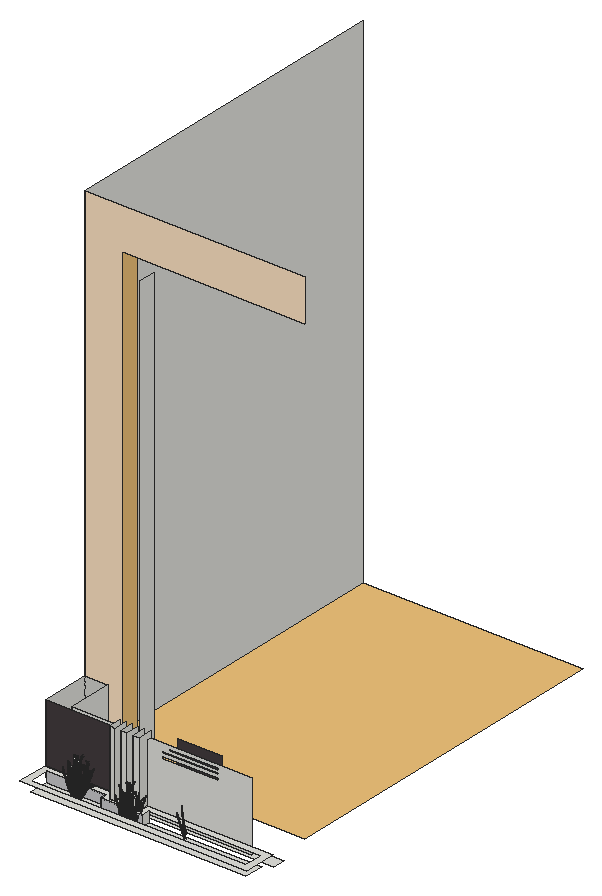
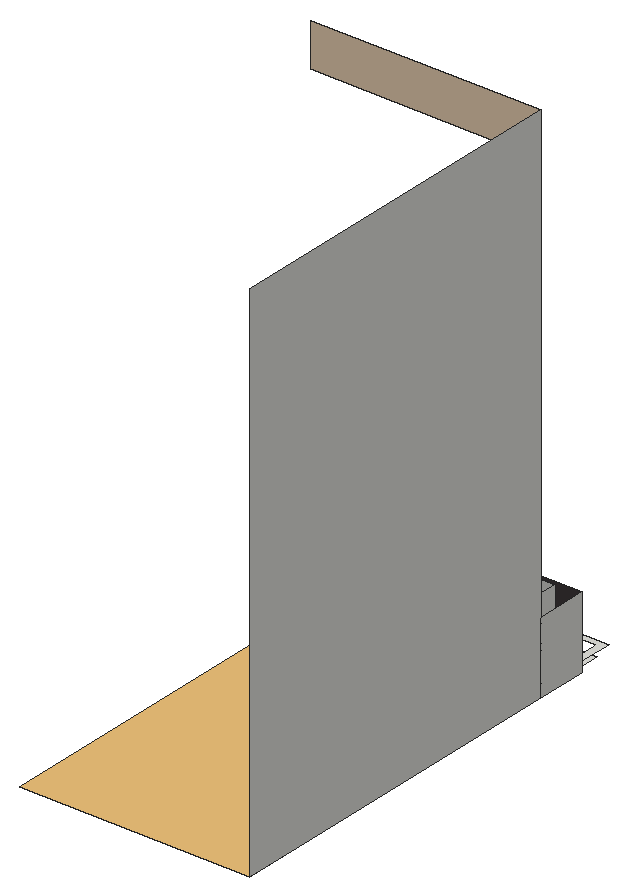
# SketchUp Ruby script. Lengths in inches.
U = 1.inch
M = Sketchup.active_model
def pt(a) = Geom::Point3d.new(a.map { |v| v * U })
def face(e, loops, mat)
  f = e.add_face(loops[0].map { |a| pt(a) })
  loops[1..].each { |l| e.add_face(l.map { |a| pt(a) }).erase! }
  f.material = f.back_material = mat if mat
  f
end
# faces: each face lists its corners as indices into pts; further lists are holes
def faces(e, pts, list, mat = nil) = list.each { |f| face(e, (f[0].is_a?(Array) ? f : [f]).map { |l| l.map { |i| pts[i] } }, mat) }
# xy, xz, yz: faces in a plane at the given z, y or x. An outline is a flat list of corners, or four numbers for a rectangle; further outlines are holes
def ring(l) = l.size == 4 ? [[l[0], l[1]], [l[2], l[1]], [l[2], l[3]], [l[0], l[3]]] : l.each_slice(2).to_a
def flat(e, list, mat, &to3) = list.each { |f| face(e, (f[0].is_a?(Array) ? f : [f]).map { |l| ring(l).map { |u, v| to3.(u, v) } }, mat) }
def xy(e, z, list, mat = nil) = flat(e, list, mat) { |x, y| [x, y, z] }
def xz(e, y, list, mat = nil) = flat(e, list, mat) { |x, z| [x, y, z] }
def yz(e, x, list, mat = nil) = flat(e, list, mat) { |y, z| [x, y, z] }
def lines(e, pts, list) = list.each { |a, b| e.add_line(pt(pts[a]), pt(pts[b])) }
# prism: a flat outline (further loops are holes) pulled along v
def prism(e, loops, v, mat = nil)
  f = face(e, loops, mat); d = Geom::Vector3d.new(v.map { |x| x * U })
  f.pushpull(f.normal.samedirection?(d) ? d.length : -d.length)
end
def box(e, o, s, mat = nil) = prism(e, [[o, [o[0] + s[0], o[1], o[2]], [o[0] + s[0], o[1] + s[1], o[2]], [o[0], o[1] + s[1], o[2]]]], [0, 0, s[2]], mat)
def at(x, y, z, deg = 0) = Geom::Transformation.translation(pt([x, y, z])) * Geom::Transformation.rotation(ORIGIN, Z_AXIS, deg.degrees)
def axes(o, x, y, z) = Geom::Transformation.new([*x, 0, *y, 0, *z, 0, *pt(o).to_a, 1])
def part(name) = M.definitions.add(name)
# library, detail: a bought-in or finely detailed component or shape, given as its bounding box
def library(name, o, s) = part(name).tap { |d| box(d.entities, o, s) }
def detail(e, o, s) = box(e.add_group.entities, o, s)
def put(e, d, t, mat = nil) = e.add_instance(d, t).tap { |i| i.material = mat if mat }
def group(e, t, mat = nil) = e.add_group.tap { |g| g.transformation = t; g.material = mat if mat }.entities
root = M.entities
M.materials.add("[0012_Bisque]").color = [255, 228, 196]
M.materials.add("[Asphalt New]").color = [67, 60, 62]
M.materials.add("[Polished Concrete New]").color = [200, 200, 203]
M.materials.add("[Wood OSB]").color = [240, 195, 122]
c1 = part("fur_instance\#8")
p = [[-0.25,1.49,0.03],[0.25,-1.49,-0.03],[0.44,-1.47,1.51],[-0.05,1.47,1.57],[0.65,-1.44,3.05],[0.16,1.45,3.11],
  [0.86,-1.42,4.59],[0.38,1.44,4.65],[1.1,-1.39,6.13],[0.62,1.43,6.18],[1.34,-1.35,7.66],[0.875,1.42,7.72],
  [1.6,-1.32,9.19],[1.14,1.41,9.25],[1.88,-1.28,10.72],[1.43,1.41,10.78],[2.18,-1.24,12.25],[1.73,1.41,12.3],
  [2.49,-1.19,13.77],[2.05,1.41,13.82],[2.83,-1.15,15.29],[2.4,1.41,15.34],[3.18,-1.09,16.8],[2.76,1.42,16.85],
  [3.56,-1.03,18.31],[3.14,1.43,18.35],[3.96,-0.97,19.81],[3.55,1.44,19.85],[4.38,-0.91,21.3],[3.99,1.46,21.35],
  [4.84,-0.83,22.78],[4.45,1.48,22.83],[5.32,-0.76,24.26],[4.93,1.51,24.31],[5.82,-0.67,25.73],[5.45,1.54,25.77],
  [6.36,-0.59,27.18],[6,1.57,27.23],[6.93,-0.49,28.625],[6.58,1.61,28.67],[7.54,-0.39,30.05],[7.19,1.66,30.1],
  [8.18,-0.28,31.47],[7.84,1.71,31.51],[8.85,-0.16,32.86],[8.53,1.77,32.9],[9.57,-0.04,34.24],[9.25,1.83,34.27],
  [10.32,0.09,35.59],[10.02,1.9,35.625],[11.12,0.23,36.92],[10.82,1.97,36.95],[11.95,0.38,38.22],[11.67,2.06,38.25],
  [12.84,0.54,39.49],[12.57,2.14,39.52],[13.76,0.71,40.73],[13.51,2.24,40.76],[14.73,0.89,41.93],[14.49,2.34,41.95],
  [15.75,1.08,43.09],[15.52,2.45,43.11],[16.82,1.28,44.2],[16.6,2.5625,44.23],[17.93,1.5,45.27],[17.73,2.68,45.29],
  [19.08,1.73,46.28],[18.9,2.81,46.3],[20.29,1.97,47.24],[20.125,2.93,47.26],[21.53,2.22,48.13],[21.39,3.0625,48.15],
  [22.82,2.5,48.96],[22.7,3.1875,48.98],[24.14,2.8125,49.72],[24.06,3.3,49.73],[25.48,3.27,50.41]]
faces(c1.entities,p,[[0,1,2,3],[3,2,4,5],[5,4,6,7],[7,6,8,9],[9,8,10,11],[11,10,12,13],[13,12,14,15],[15,14,16,17],
  [17,16,18,19],[19,18,20,21],[21,20,22,23],[23,22,24,25],[25,24,26,27],[27,26,28,29],[29,28,30,31],[31,30,32,33],
  [33,32,34,35],[35,34,36,37],[37,36,38,39],[39,38,40,41],[41,40,42,43],[43,42,44,45],[45,44,46,47],[47,46,48,49],
  [49,48,50,51],[51,50,52,53],[53,52,54,55],[55,54,56,57],[57,56,58,59],[59,58,60,61],[61,60,62,63],[63,62,64,65],
  [65,64,66,67],[67,66,68,69],[69,68,70,71],[71,70,72,73],[73,72,74,75],[75,74,76]])
xy(root,0,[[11.52,60.29,230.42,60.29,230.42,79.88,115.35,79.88,115.35,73.19,72.16,73.19,72.16,79.88,11.52,79.88],[78.43,76.52,84.2,86.15],[89.84,76.52,96.33,86.15],[102.45,76.52,109.08,86.15],[5.25,86.15,238.24,86.15,238.24,98.26,211.95,98.26,211.95,90.32,28.64,90.32,28.64,136.77,5.25,136.77],
  [43.27,136.77,60.84,154.83]])
xy(root,0,[[5.25,136.77,43.27,136.77,43.27,154.83,60.84,154.83,60.84,136.77,228.75,136.77,228.75,490.875,5.25,490.875]],"[Wood OSB]")
xy(root,10.375,[[[5.25,54.02,236.6875,54.02,236.6875,86.15,109.08,86.15,109.08,76.52,102.45,76.52,102.45,86.15,96.33,86.15,96.33,76.52,89.84,76.52,89.84,86.15,84.2,86.15,84.2,76.52,78.43,76.52,78.43,86.15,5.25,86.15],[11.52,60.29,11.52,79.88,72.16,79.88,72.16,73.19,115.35,73.19,115.35,79.88,230.42,79.88,230.42,60.29]]])
xz(root,73.19,[[72.16,0,90.47,10.375],[90.47,0,102.6,10.375],[102.6,0,115.35,10.375]],"[Polished Concrete New]")
xz(root,76.52,[[78.43,0,84.2,10.375],[89.84,0,96.33,10.375],[102.45,0,109.08,10.375],[78.43,10.375,84.2,76.5625],[89.84,10.375,96.33,76.5625],
  [102.45,10.375,109.08,76.5625]])
xz(root,79.88,[[11.52,0,72.16,10.375]],"[Polished Concrete New]")
xz(root,86.15,[[5.25,0,78.43,10.375],[84.2,0,89.84,10.375],[96.33,0,102.45,10.375]])
xz(root,86.15,[[5.25,10.375,78.43,70.5625],[84.2,10.375,89.84,70.5625],[96.33,10.375,102.45,70.5625]],"[Asphalt New]")
xz(root,90.32,[[[28.64,0,211.95,70.5625],[120.75,55.78,178.5,58.72],[120.5,60.82,178.5,63.13],[127.31,64.89,178.5,67.33]]])
xz(root,136.77,[[28.64,0,43.27,0,43.27,470.41,228.75,470.41,228.75,513.13,5.25,513.13,5.25,70.5625,28.64,70.5625]],"[0012_Bisque]")
xz(root,136.77,[[99.93,0,144.79,46.08]],"[Asphalt New]")
yz(root,5.25,[[86.15,0,136.77,70.5625],[136.77,0,490.875,513.13]])
yz(root,28.64,[[90.32,0,136.77,70.5625]])
yz(root,43.27,[[136.77,0,154.83,470.41]],"[Wood OSB]")
yz(root,60.84,[[136.77,0,154.83,450.1]])
yz(root,72.16,[[73.19,0,79.88,10.375]])
yz(root,78.43,[[76.52,0,86.15,10.375],[76.52,10.375,76.52,76.5625,90.09,76.5625,90.09,70.5625,86.15,70.5625,86.15,10.375]])
yz(root,84.2,[[76.52,0,86.15,10.375],[76.52,10.375,86.15,10.375,86.15,70.5625,90.09,70.5625,90.09,76.5625,76.52,76.5625]])
yz(root,89.84,[[76.52,0,86.15,10.375],[76.52,10.375,76.52,76.5625,90.32,76.5625,90.32,70.5625,86.15,70.5625,86.15,10.375]])
yz(root,96.33,[[76.52,0,86.15,10.375],[76.52,10.375,86.15,10.375,86.15,70.5625,90.32,70.5625,90.32,76.5625,76.52,76.5625]])
yz(root,102.45,[[76.52,0,86.15,10.375],[76.52,10.375,76.52,76.5625,90.32,76.5625,90.32,70.5625,86.15,70.5625,86.15,10.375]])
yz(root,109.08,[[76.52,0,86.15,10.375],[76.52,10.375,86.15,10.375,86.15,70.5625,90.32,70.5625,90.32,76.5625,76.52,76.5625]])
yz(root,115.35,[[73.19,0,79.88,10.375]])
put(root,c1,axes([98.37,74.84,2.3],[-0.12046,-0.19753,0.07695],[0.20061,-0.12871,0.24478],[-0.08711,0.03599,0.49657]))
put(root,c1,axes([44.62,71.44,4.95],[0.17949,0.03208,0.20009],[-0.02216,0.19765,-0.22548],[-0.11594,0.04484,0.37468]))
put(root,c1,axes([97.88,71.44,-0.97],[0.17949,0.03208,0.20009],[-0.02216,0.19765,-0.22548],[-0.11594,0.04484,0.37468]))
put(root,c1,axes([48.35,71.48,11.67],[-0.12955,0.21354,-0.0433],[-0.21401,-0.10243,0.0018],[-0.01549,-0.03509,0.55942]))
put(root,c1,axes([101.61,71.48,5.75],[-0.12955,0.21354,-0.0433],[-0.21401,-0.10243,0.0018],[-0.01549,-0.03509,0.55942]))
put(root,c1,axes([46.31,70.35,7.49],[0.00664,0.20286,-0.1262],[-0.19518,0.01818,-0.18229],[-0.08769,0.01816,0.42485]))
put(root,c1,axes([99.5625,70.35,1.57],[0.00664,0.20286,-0.1262],[-0.19518,0.01818,-0.18229],[-0.08769,0.01816,0.42485]))
put(root,c1,axes([48.88,72.47,3.5],[0.03807,-0.14827,0.33406],[0.19165,0.02974,-0.03379],[-0.02912,0.11286,0.28781]))
put(root,c1,axes([102.14,72.47,-2.42],[0.03807,-0.14827,0.33406],[0.19165,0.02974,-0.03379],[-0.02912,0.11286,0.28781]))
put(root,c1,axes([47.29,69.77,2.75],[0.10395,0.11836,-0.12851],[-0.11439,0.07411,-0.26217],[-0.07351,0.08501,0.2481]))
put(root,c1,axes([100.55,69.77,-3.17],[0.10395,0.11836,-0.12851],[-0.11439,0.07411,-0.26217],[-0.07351,0.08501,0.2481]))
put(root,c1,axes([41.98,71.41,6.21],[-0.08139,0.23064,-0.15312],[-0.1699,-0.05496,-0.32193],[-0.16391,-0.02606,0.43057]))
put(root,c1,axes([95.24,71.41,0.29],[-0.08139,0.23064,-0.15312],[-0.1699,-0.05496,-0.32193],[-0.16391,-0.02606,0.43057]))
put(root,c1,axes([158.29,71.41,5.67],[-0.08139,0.23064,-0.15312],[-0.1699,-0.05496,-0.32193],[-0.16391,-0.02606,0.43057]))
put(root,c1,axes([46.52,72.15,2.91],[0.12897,-0.08882,0.30598],[0.12311,0.13439,-0.14076],[-0.0848,0.09806,0.28618]))
put(root,c1,axes([99.78,72.15,-3.01],[0.12897,-0.08882,0.30598],[0.12311,0.13439,-0.14076],[-0.0848,0.09806,0.28618]))
put(root,c1,axes([52.9,72.82,3.01],[-0.12598,-0.09298,0.35138],[0.14548,-0.16001,0.09177],[0.09178,0.08501,0.30971]))
put(root,c1,axes([106.16,72.82,-2.91],[-0.12598,-0.09298,0.35138],[0.14548,-0.16001,0.09177],[0.09178,0.08501,0.30971]))
put(root,c1,axes([52.3,74.05,6],[0.17475,-0.1628,0.03799],[0.13362,0.1403,-0.32315],[0.08136,0.06328,0.41208]))
put(root,c1,axes([105.55,74.05,0.08],[0.17475,-0.1628,0.03799],[0.13362,0.1403,-0.32315],[0.08136,0.06328,0.41208]))
put(root,c1,axes([51.24,73.21,2.9],[-0.04728,-0.14736,0.35137],[0.1919,-0.08682,-0.02284],[0.06183,0.09936,0.30152]))
put(root,c1,axes([104.5,73.21,-3.02],[-0.04728,-0.14736,0.35137],[0.1919,-0.08682,-0.02284],[0.06183,0.09936,0.30152]))
put(root,c1,axes([52.5,74.19,5.44],[-0.12567,-0.14648,0.32324],[0.17955,-0.15616,0.02426],[0.08105,0.06304,0.41053]))
put(root,c1,axes([105.76,74.19,-0.48],[-0.12567,-0.14648,0.32324],[0.17955,-0.15616,0.02426],[0.08105,0.06304,0.41053]))
put(root,c1,axes([53.38,70.52,3.8],[-0.05675,0.18901,-0.12396],[-0.14509,-0.01855,0.32364],[0.12915,0.03597,0.29172]))
put(root,c1,axes([106.64,70.52,-2.12],[-0.05675,0.18901,-0.12396],[-0.14509,-0.01855,0.32364],[0.12915,0.03597,0.29172]))
put(root,c1,axes([45.94,73.15,3.77],[0.03058,-0.16302,0.35291],[0.18885,0.05742,0.07777],[-0.09099,0.10522,0.30707]))
put(root,c1,axes([99.2,73.15,-2.15],[0.03058,-0.16302,0.35291],[0.18885,0.05742,0.07777],[-0.09099,0.10522,0.30707]))
put(root,c1,axes([50.43,72.07,11.08],[-0.19584,0.16179,-0.00169],[-0.1515,-0.17581,0.15196],[0.03573,-0.00363,0.539]))
put(root,c1,axes([103.69,72.07,5.16],[-0.19584,0.16179,-0.00169],[-0.1515,-0.17581,0.15196],[0.03573,-0.00363,0.539]))
put(root,c1,axes([46.46,70.35,3.21],[0.12204,0.11956,-0.03437],[-0.09323,0.10261,-0.31254],[-0.10097,0.07745,0.26536]))
put(root,c1,axes([99.72,70.35,-2.71],[0.12204,0.11956,-0.03437],[-0.09323,0.10261,-0.31254],[-0.10097,0.07745,0.26536]))
put(root,c1,axes([50.18,71.18,8.72],[0.03623,0.20627,-0.12936],[-0.21911,0.05324,0.03667],[0.02079,0.00357,0.48088]))
put(root,c1,axes([103.4375,71.18,2.8],[0.03623,0.20627,-0.12936],[-0.21911,0.05324,0.03667],[0.02079,0.00357,0.48088]))
put(root,c1,axes([46.1,72.88,7.66],[0.2158,0.0049,0.14651],[-0.01279,0.21776,-0.18636],[-0.08047,0.03325,0.45875]))
put(root,c1,axes([99.36,72.88,1.74],[0.2158,0.0049,0.14651],[-0.01279,0.21776,-0.18636],[-0.08047,0.03325,0.45875]))
put(root,c1,axes([47.74,70.84,4.39],[-0.12886,0.11444,-0.22997],[-0.12949,-0.11784,0.12414],[-0.04678,0.07389,0.33152]))
put(root,c1,axes([101,70.84,-1.53],[-0.12886,0.11444,-0.22997],[-0.12949,-0.11784,0.12414],[-0.04678,0.07389,0.33152]))
put(root,c1,axes([49.2,71.02,3.48],[0.17646,0.02205,-0.09309],[-0.04854,0.13883,-0.29657],[0.00073,0.10392,0.26687]))
put(root,c1,axes([102.46,71.02,-2.44],[0.17646,0.02205,-0.09309],[-0.04854,0.13883,-0.29657],[0.00073,0.10392,0.26687]))
put(root,c1,axes([49.08,72.23,12.43],[0.11288,0.21144,-0.04258],[-0.23471,0.1258,-0.00774],[-0.00125,-0.03681,0.58142]))
put(root,c1,axes([102.34,72.23,6.51],[0.11288,0.21144,-0.04258],[-0.23471,0.1258,-0.00774],[-0.00125,-0.03681,0.58142]))
put(root,c1,axes([43.09,71.5,5.32],[0.05993,0.19956,0.02934],[-0.16765,0.09615,-0.32784],[-0.14862,0.00196,0.40149]))
put(root,c1,axes([96.35,71.5,-0.6],[0.05993,0.19956,0.02934],[-0.16765,0.09615,-0.32784],[-0.14862,0.00196,0.40149]))
put(root,c1,axes([48.34,71.8,9.77],[-0.15948,0.17543,-0.11844],[-0.17074,-0.13846,0.07646],[-0.0175,0.01182,0.50519]))
put(root,c1,axes([101.6,71.8,3.85],[-0.15948,0.17543,-0.11844],[-0.17074,-0.13846,0.07646],[-0.0175,0.01182,0.50519]))
put(root,c1,axes([52.93,70.62,2.85],[-0.02741,0.17392,-0.23076],[-0.16029,0.02766,0.23757],[0.10574,0.05755,0.28081]))
put(root,c1,axes([106.1875,70.62,-3.07],[-0.02741,0.17392,-0.23076],[-0.16029,0.02766,0.23757],[0.10574,0.05755,0.28081]))
put(root,c1,axes([49.28,73.07,11.15],[-0.22966,0.11975,-0.02971],[-0.1055,-0.20961,0.14888],[0.00986,0.00949,0.54546]))
put(root,c1,axes([102.54,73.07,5.23],[-0.22966,0.11975,-0.02971],[-0.1055,-0.20961,0.14888],[0.00986,0.00949,0.54546]))
put(root,c1,axes([45.28,71.875,5.21],[0.149,0.11824,0.07488],[-0.1012,0.16059,-0.29075],[-0.11547,0.04466,0.37315]))
put(root,c1,axes([98.54,71.875,-0.71],[0.149,0.11824,0.07488],[-0.1012,0.16059,-0.29075],[-0.11547,0.04466,0.37315]))
put(root,c1,axes([43.54,71.44,3.95],[-0.06018,0.17755,-0.31983],[-0.13865,-0.10086,-0.20049],[-0.15862,0.04585,0.31318]))
put(root,c1,axes([96.8,71.44,-1.97],[-0.06018,0.17755,-0.31983],[-0.13865,-0.10086,-0.20049],[-0.15862,0.04585,0.31318]))
put(root,c1,axes([159.85,71.44,3.41],[-0.06018,0.17755,-0.31983],[-0.13865,-0.10086,-0.20049],[-0.15862,0.04585,0.31318]))
put(root,c1,axes([43.11,72.31,8.17],[-0.04995,0.23864,-0.11124],[-0.21419,-0.02204,-0.24055],[-0.12191,-0.01612,0.49664]))
put(root,c1,axes([96.37,72.31,2.25],[-0.04995,0.23864,-0.11124],[-0.21419,-0.02204,-0.24055],[-0.12191,-0.01612,0.49664]))
put(root,c1,axes([159.42,72.31,7.63],[-0.04995,0.23864,-0.11124],[-0.21419,-0.02204,-0.24055],[-0.12191,-0.01612,0.49664]))
put(root,c1,axes([45.58,71.77,3.69],[-0.12441,0.08913,-0.33358],[-0.11522,-0.1494,0.09624],[-0.1115,0.08552,0.29301]))
put(root,c1,axes([98.84,71.77,-2.23],[-0.12441,0.08913,-0.33358],[-0.11522,-0.1494,0.09624],[-0.1115,0.08552,0.29301]))
put(root,c1,axes([53.68,72.21,8.09],[0.06433,0.21786,-0.19116],[-0.21809,0.08663,0.16557],[0.09246,-0.00116,0.48782]))
put(root,c1,axes([106.9375,72.21,2.17],[0.06433,0.21786,-0.19116],[-0.21809,0.08663,0.16557],[0.09246,-0.00116,0.48782]))
put(root,c1,axes([53.28,73.11,3.76],[-0.18323,0.03397,0.2678],[0.02904,-0.19802,0.26654],[0.12063,0.06566,0.32036]))
put(root,c1,axes([106.54,73.11,-2.16],[-0.18323,0.03397,0.2678],[0.02904,-0.19802,0.26654],[0.12063,0.06566,0.32036]))
put(root,c1,axes([47.75,71.89,5.58],[-0.16185,0.10098,-0.22361],[-0.11509,-0.14728,0.17524],[-0.05085,0.08033,0.3604]))
put(root,c1,axes([101,71.89,-0.34],[-0.16185,0.10098,-0.22361],[-0.11509,-0.14728,0.17524],[-0.05085,0.08033,0.3604]))
put(root,c1,axes([50,71.96,6.56],[-0.1319,0.16634,-0.13442],[-0.16484,-0.10583,0.16664],[0.0172,0.04548,0.42308]))
put(root,c1,axes([103.26,71.96,0.64],[-0.1319,0.16634,-0.13442],[-0.16484,-0.10583,0.16664],[0.0172,0.04548,0.42308]))
put(root,c1,axes([49.93,72.08,4.26],[0.16157,0.07757,-0.19831],[-0.11325,0.15562,-0.18994],[0.0239,0.07619,0.35007]))
put(root,c1,axes([103.19,72.08,-1.66],[0.16157,0.07757,-0.19831],[-0.11325,0.15562,-0.18994],[0.0239,0.07619,0.35007]))
put(root,c1,axes([47.79,72.54,4.77],[-0.18808,0.05687,-0.16759],[-0.06647,-0.17012,0.23097],[-0.05108,0.08069,0.36201]))
put(root,c1,axes([101.05,72.54,-1.15],[-0.18808,0.05687,-0.16759],[-0.06647,-0.17012,0.23097],[-0.05108,0.08069,0.36201]))
put(root,c1,axes([49.55,71.66,3.26],[-0.17438,0.07052,-0.11324],[-0.07295,-0.12692,0.30042],[0.00076,0.10733,0.27565]))
put(root,c1,axes([102.8,71.66,-2.66],[-0.17438,0.07052,-0.11324],[-0.07295,-0.12692,0.30042],[0.00076,0.10733,0.27565]))
put(root,c1,axes([42.98,73.21,3],[0.15352,0.06911,0.26676],[-0.03494,0.20117,-0.28887],[-0.16523,0.04776,0.32623]))
put(root,c1,axes([96.24,73.21,-2.92],[0.15352,0.06911,0.26676],[-0.03494,0.20117,-0.28887],[-0.16523,0.04776,0.32623]))
put(root,c1,axes([48.83,73.51,5.75],[-0.21697,-0.00618,0.04885],[0.02773,-0.18874,0.29817],[-0.00075,0.0894,0.38532]))
put(root,c1,axes([102.09,73.51,-0.16],[-0.21697,-0.00618,0.04885],[0.02773,-0.18874,0.29817],[-0.00075,0.0894,0.38532]))
put(root,c1,axes([51.36,72.27,8.77],[0.08086,0.19655,-0.23287],[-0.213,0.10459,0.05528],[0.05877,0.03065,0.4692]))
put(root,c1,axes([104.62,72.27,2.85],[0.08086,0.19655,-0.23287],[-0.213,0.10459,0.05528],[0.05877,0.03065,0.4692]))
put(root,c1,axes([44.09,72.72,8.49],[-0.0789,0.22714,-0.18379],[-0.20548,-0.06456,-0.18143],[-0.11262,0.00359,0.48952]))
put(root,c1,axes([97.35,72.72,2.57],[-0.0789,0.22714,-0.18379],[-0.20548,-0.06456,-0.18143],[-0.11262,0.00359,0.48952]))
put(root,c1,axes([50.23,74.67,5.11],[-0.18748,-0.08453,0.22152],[0.12512,-0.17975,0.22209],[0.0273,0.08703,0.39989]))
put(root,c1,axes([103.49,74.67,-0.8],[-0.18748,-0.08453,0.22152],[0.12512,-0.17975,0.22209],[0.0273,0.08703,0.39989]))
put(root,c1,axes([51.65,71.4,3.21],[0.02265,0.14627,-0.32338],[-0.18321,0.06424,0.06],[0.05776,0.09281,0.28164]))
put(root,c1,axes([104.91,71.4,-2.71],[0.02265,0.14627,-0.32338],[-0.18321,0.06424,0.06],[0.05776,0.09281,0.28164]))
put(root,c1,axes([52.62,72.78,10.375],[-0.06671,0.24175,-0.07521],[-0.22931,-0.04686,0.25475],[0.09711,-0.00122,0.51237]))
put(root,c1,axes([105.88,72.78,4.46],[-0.06671,0.24175,-0.07521],[-0.22931,-0.04686,0.25475],[0.09711,-0.00122,0.51237]))
put(root,c1,axes([47.21,72.73,10.92],[-0.03892,0.23857,-0.13916],[-0.24331,-0.01786,-0.06409],[-0.04532,0.0056,0.5395]))
put(root,c1,axes([100.47,72.73,5],[-0.03892,0.23857,-0.13916],[-0.24331,-0.01786,-0.06409],[-0.04532,0.0056,0.5395]))
put(root,c1,axes([48.33,72.03,6.05],[0.14274,0.1248,-0.18106],[-0.14873,0.12853,-0.2232],[-0.02656,0.08555,0.36591]))
put(root,c1,axes([101.59,72.03,0.13],[0.14274,0.1248,-0.18106],[-0.14873,0.12853,-0.2232],[-0.02656,0.08555,0.36591]))
put(root,c1,axes([47.45,72.71,7.34],[0.14854,0.14611,-0.10639],[-0.16099,0.14725,-0.20019],[-0.04301,0.04934,0.44533]))
put(root,c1,axes([100.71,72.71,1.42],[0.14854,0.14611,-0.10639],[-0.16099,0.14725,-0.20019],[-0.04301,0.04934,0.44533]))
put(root,c1,axes([45.02,74.08,7.62],[0.21224,0.07306,0.08848],[-0.08036,0.21667,-0.23259],[-0.08448,0.0349,0.48158]))
put(root,c1,axes([98.28,74.08,1.7],[0.21224,0.07306,0.08848],[-0.08036,0.21667,-0.23259],[-0.08448,0.0349,0.48158]))
put(root,c1,axes([45.07,73.15,2.71],[-0.14657,0.06865,-0.32949],[-0.09952,-0.16829,0.15169],[-0.11649,0.08935,0.30613]))
put(root,c1,axes([98.33,73.15,-3.21],[-0.14657,0.06865,-0.32949],[-0.09952,-0.16829,0.15169],[-0.11649,0.08935,0.30613]))
put(root,c1,axes([47.55,73.3,10.12],[0.10044,0.20522,-0.10286],[-0.22219,0.11383,-0.10772],[-0.03192,0.01018,0.52996]))
put(root,c1,axes([100.8125,73.3,4.2],[0.10044,0.20522,-0.10286],[-0.22219,0.11383,-0.10772],[-0.03192,0.01018,0.52996]))
put(root,c1,axes([47.7,73.95,11.55],[0.19334,0.14897,-0.05271],[-0.17118,0.19893,-0.14866],[-0.0338,0.01079,0.56126]))
put(root,c1,axes([100.96,73.95,5.63],[0.19334,0.14897,-0.05271],[-0.17118,0.19893,-0.14866],[-0.0338,0.01079,0.56126]))
put(root,c1,axes([52.84,73.23,8.09],[-0.1067,0.21804,-0.07354],[-0.20586,-0.08261,0.23931],[0.07827,0.01663,0.48727]))
put(root,c1,axes([106.1,73.23,2.17],[-0.1067,0.21804,-0.07354],[-0.20586,-0.08261,0.23931],[0.07827,0.01663,0.48727]))
put(root,c1,axes([44.42,72.97,6.33],[-0.09952,0.18231,-0.31022],[-0.16857,-0.11721,-0.10121],[-0.1255,0.04853,0.40556]))
put(root,c1,axes([97.68,72.97,0.41],[-0.09952,0.18231,-0.31022],[-0.16857,-0.11721,-0.10121],[-0.1255,0.04853,0.40556]))
put(root,c1,axes([49.84,73.26,2.71],[0.19789,0.01674,-0.08664],[-0.04397,0.1548,-0.33323],[0.00081,0.11511,0.29561]))
put(root,c1,axes([103.1,73.26,-3.21],[0.19789,0.01674,-0.08664],[-0.04397,0.1548,-0.33323],[0.00081,0.11511,0.29561]))
put(root,c1,axes([51.63,73.73,3.62],[0.19779,0.00085,-0.20861],[-0.06023,0.17892,-0.30359],[0.06469,0.10395,0.31543]))
put(root,c1,axes([104.89,73.73,-2.3],[0.19779,0.00085,-0.20861],[-0.06023,0.17892,-0.30359],[0.06469,0.10395,0.31543]))
put(root,c1,axes([46.71,73.32,2.82],[-0.17971,0.05049,-0.21333],[-0.08082,-0.15328,0.27859],[-0.06056,0.11282,0.29972]))
put(root,c1,axes([99.97,73.32,-3.1],[-0.17971,0.05049,-0.21333],[-0.08082,-0.15328,0.27859],[-0.06056,0.11282,0.29972]))
put(root,c1,axes([51.9,73.24,9.89],[-0.0236,0.24008,-0.16159],[-0.23761,0.00409,0.20091],[0.0806,0.01712,0.5018]))
put(root,c1,axes([105.16,73.24,3.97],[-0.0236,0.24008,-0.16159],[-0.23761,0.00409,0.20091],[0.0806,0.01712,0.5018]))
put(root,c1,axes([47.68,73.01,8.65],[-0.03105,0.21618,-0.23248],[-0.22713,-0.0199,-0.04743],[-0.04502,0.05164,0.46606]))
put(root,c1,axes([100.94,73.01,2.74],[-0.03105,0.21618,-0.23248],[-0.22713,-0.0199,-0.04743],[-0.04502,0.05164,0.46606]))
put(root,c1,axes([49.67,73.29,4.3],[-0.13558,0.14856,-0.21429],[-0.16001,-0.10351,0.19496],[-0.00072,0.08572,0.36945]))
put(root,c1,axes([102.93,73.29,-1.625],[-0.13558,0.14856,-0.21429],[-0.16001,-0.10351,0.19496],[-0.00072,0.08572,0.36945]))
put(root,c1,axes([46.5,74.14,9.3125],[-0.1589,0.17803,-0.2479],[-0.17756,-0.14881,0.0508],[-0.06832,0.04712,0.49383]))
put(root,c1,axes([99.76,74.14,3.39],[-0.1589,0.17803,-0.2479],[-0.17756,-0.14881,0.0508],[-0.06832,0.04712,0.49383]))
put(root,c1,axes([47.13,73.78,3.85],[0.1975,0.05806,-0.0072],[-0.05058,0.15655,-0.36297],[-0.06266,0.11673,0.31011]))
put(root,c1,axes([100.39,73.78,-2.07],[0.1975,0.05806,-0.0072],[-0.05058,0.15655,-0.36297],[-0.06266,0.11673,0.31011]))
put(root,c1,axes([45.03,75.29,4.34],[0.19488,-0.04118,0.27862],[0.0814,0.18631,-0.28554],[-0.10045,0.11615,0.33899]))
put(root,c1,axes([98.29,75.29,-1.58],[0.19488,-0.04118,0.27862],[0.0814,0.18631,-0.28554],[-0.10045,0.11615,0.33899]))
put(root,c1,axes([47.1875,73.25,3.34],[-0.05838,0.1486,-0.35065],[-0.18856,-0.06365,0.02437],[-0.06066,0.11302,0.30025]))
put(root,c1,axes([100.44,73.25,-2.57],[-0.05838,0.1486,-0.35065],[-0.18856,-0.06365,0.02437],[-0.06066,0.11302,0.30025]))
put(root,c1,axes([54.61,74.49,7.17],[-0.08095,0.24089,-0.09572],[-0.20653,-0.05261,0.34972],[0.13417,0.02289,0.45313]))
put(root,c1,axes([107.87,74.49,1.25],[-0.08095,0.24089,-0.09572],[-0.20653,-0.05261,0.34972],[0.13417,0.02289,0.45313]))
put(root,c1,axes([47.03,78.21,5.8],[0.05792,-0.21665,0.35228],[0.2474,0.04272,-0.03732],[-0.03274,0.10545,0.45101]))
put(root,c1,axes([100.29,78.21,-0.12],[0.05792,-0.21665,0.35228],[0.2474,0.04272,-0.03732],[-0.03274,0.10545,0.45101]))
put(root,c1,axes([49.55,77.59,5.42],[0.18259,-0.1619,0.22728],[0.17109,0.14301,-0.26039],[-0.00086,0.10227,0.44077]))
put(root,c1,axes([102.81,77.59,-0.5],[0.18259,-0.1619,0.22728],[0.17109,0.14301,-0.26039],[-0.00086,0.10227,0.44077]))
put(root,c1,axes([46.23,74.33,7.76],[0.04781,0.21803,-0.18144],[-0.22564,0.05394,-0.16456],[-0.06613,0.04562,0.47803]))
put(root,c1,axes([99.49,74.33,1.84],[0.04781,0.21803,-0.18144],[-0.22564,0.05394,-0.16456],[-0.06613,0.04562,0.47803]))
put(root,c1,axes([53.2,76.41,5.43],[-0.23752,0.04727,0.17981],[0.00037,-0.22718,0.3018],[0.08784,0.06833,0.44492]))
put(root,c1,axes([106.46,76.41,-0.49],[-0.23752,0.04727,0.17981],[0.00037,-0.22718,0.3018],[0.08784,0.06833,0.44492]))
put(root,c1,axes([45.02,75.91,4.91],[0.22314,0.03503,0.11397],[-0.0252,0.21097,-0.3146],[-0.08653,0.08429,0.4222]))
put(root,c1,axes([98.28,75.91,-1.01],[0.22314,0.03503,0.11397],[-0.0252,0.21097,-0.3146],[-0.08653,0.08429,0.4222]))
put(root,c1,axes([47.96,77.82,5.9],[-0.20442,-0.12057,0.16665],[0.14603,-0.18202,0.30806],[-0.03237,0.10426,0.44592]))
put(root,c1,axes([101.22,77.82,-0.02],[-0.20442,-0.12057,0.16665],[0.14603,-0.18202,0.30806],[-0.03237,0.10426,0.44592]))
put(root,c1,axes([50.5,74.13,4.07],[-0.15443,0.14355,-0.21021],[-0.15015,-0.09516,0.30489],[0.0337,0.11705,0.31784]))
put(root,c1,axes([103.76,74.13,-1.85],[-0.15443,0.14355,-0.21021],[-0.15015,-0.09516,0.30489],[0.0337,0.11705,0.31784]))
put(root,c1,axes([48.14,74.42,3.15],[-0.08555,0.15021,-0.34626],[-0.19424,-0.0665,0.11459],[-0.03163,0.1226,0.31264]))
put(root,c1,axes([101.4,74.42,-2.77],[-0.08555,0.15021,-0.34626],[-0.19424,-0.0665,0.11459],[-0.03163,0.1226,0.31264]))
put(root,c1,axes([45.86,76.73,7.78],[-0.18658,0.14503,-0.30144],[-0.1645,-0.17028,0.18908],[-0.06369,0.10062,0.4514]))
put(root,c1,axes([99.12,76.73,1.86],[-0.18658,0.14503,-0.30144],[-0.1645,-0.17028,0.18908],[-0.06369,0.10062,0.4514]))
put(root,c1,axes([50.35,77.37,5.12],[-0.22222,0.12257,-0.08636],[-0.10729,-0.17964,0.33239],[0.02989,0.09528,0.43781]))
put(root,c1,axes([103.61,77.37,-0.8],[-0.22222,0.12257,-0.08636],[-0.10729,-0.17964,0.33239],[0.02989,0.09528,0.43781]))
put(root,c1,axes([49.55,76.54,7.76],[0.16049,0.15534,-0.27829],[-0.19592,0.15388,-0.21201],[-0.00087,0.10351,0.44615]))
put(root,c1,axes([102.81,76.54,1.84],[0.16049,0.15534,-0.27829],[-0.19592,0.15388,-0.21201],[-0.00087,0.10351,0.44615]))
put(root,c1,axes([50.73,78.43,5.28],[-0.24957,0.08322,-0.01695],[-0.05226,-0.18613,0.43808],[0.0399,0.13857,0.37627]))
put(root,c1,axes([103.99,78.43,-0.64],[-0.24957,0.08322,-0.01695],[-0.05226,-0.18613,0.43808],[0.0399,0.13857,0.37627]))
